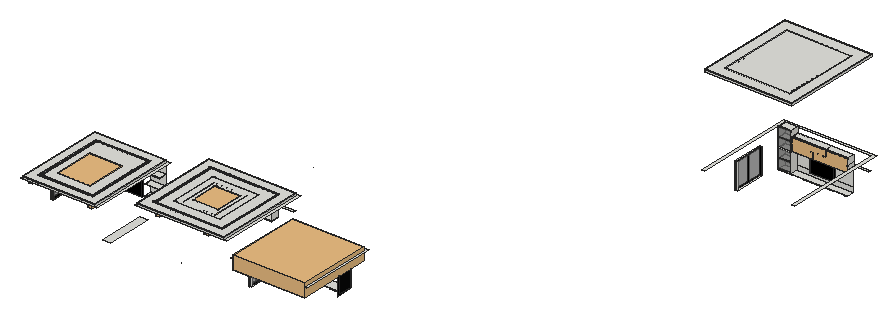
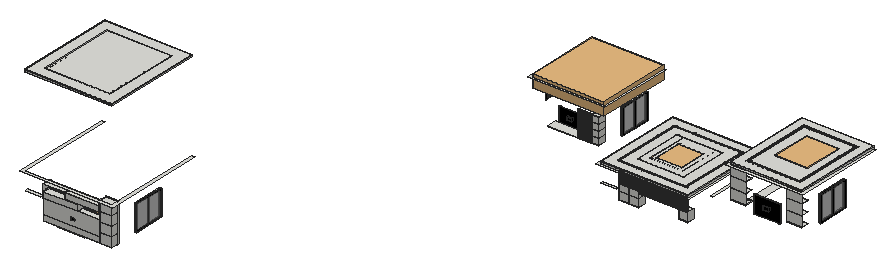
# SketchUp Ruby script. Lengths in inches.
U = 1.inch
M = Sketchup.active_model
def pt(a) = Geom::Point3d.new(a.map { |v| v * U })
def face(e, loops, mat)
  f = e.add_face(loops[0].map { |a| pt(a) })
  loops[1..].each { |l| e.add_face(l.map { |a| pt(a) }).erase! }
  f.material = f.back_material = mat if mat
  f
end
# faces: each face lists its corners as indices into pts; further lists are holes
def faces(e, pts, list, mat = nil) = list.each { |f| face(e, (f[0].is_a?(Array) ? f : [f]).map { |l| l.map { |i| pts[i] } }, mat) }
# xy, xz, yz: faces in a plane at the given z, y or x. An outline is a flat list of corners, or four numbers for a rectangle; further outlines are holes
def ring(l) = l.size == 4 ? [[l[0], l[1]], [l[2], l[1]], [l[2], l[3]], [l[0], l[3]]] : l.each_slice(2).to_a
def flat(e, list, mat, &to3) = list.each { |f| face(e, (f[0].is_a?(Array) ? f : [f]).map { |l| ring(l).map { |u, v| to3.(u, v) } }, mat) }
def xy(e, z, list, mat = nil) = flat(e, list, mat) { |x, y| [x, y, z] }
def xz(e, y, list, mat = nil) = flat(e, list, mat) { |x, z| [x, y, z] }
def yz(e, x, list, mat = nil) = flat(e, list, mat) { |y, z| [x, y, z] }
def lines(e, pts, list) = list.each { |a, b| e.add_line(pt(pts[a]), pt(pts[b])) }
# prism: a flat outline (further loops are holes) pulled along v
def prism(e, loops, v, mat = nil)
  f = face(e, loops, mat); d = Geom::Vector3d.new(v.map { |x| x * U })
  f.pushpull(f.normal.samedirection?(d) ? d.length : -d.length)
end
def box(e, o, s, mat = nil) = prism(e, [[o, [o[0] + s[0], o[1], o[2]], [o[0] + s[0], o[1] + s[1], o[2]], [o[0], o[1] + s[1], o[2]]]], [0, 0, s[2]], mat)
def at(x, y, z, deg = 0) = Geom::Transformation.translation(pt([x, y, z])) * Geom::Transformation.rotation(ORIGIN, Z_AXIS, deg.degrees)
def axes(o, x, y, z) = Geom::Transformation.new([*x, 0, *y, 0, *z, 0, *pt(o).to_a, 1])
def part(name) = M.definitions.add(name)
# library, detail: a bought-in or finely detailed component or shape, given as its bounding box
def library(name, o, s) = part(name).tap { |d| box(d.entities, o, s) }
def detail(e, o, s) = box(e.add_group.entities, o, s)
def put(e, d, t, mat = nil) = e.add_instance(d, t).tap { |i| i.material = mat if mat }
def group(e, t, mat = nil) = e.add_group.tap { |g| g.transformation = t; g.material = mat if mat }.entities
root = M.entities
M.materials.add("Chrome_Polished").color = [2, 2, 2]
M.materials.add("Plastic_Metalic_Black").color = [8, 8, 8]
M.materials.add("[0137_Black]").color = [0, 0, 0]
M.materials.add("[Color M00]1").color = [254, 254, 254]
M.materials.add("[Color_008]").color = [30, 30, 30]
M.materials.add("[Color_009]").color = [0, 0, 0]
M.materials.add("[Color_D14]").color = [173, 154, 131]
M.materials.add("[Translucent Glass Gray]1").color = [128, 128, 128]
M.materials["[Translucent Glass Gray]1"].alpha = 0.5
M.materials.add("[Translucent_Glass_Gray]").color = [128, 128, 128]
M.materials["[Translucent_Glass_Gray]"].alpha = 0.5
M.materials.add("blackened steel1").color = [30, 30, 30]
c1 = library("SKT_Nearly Natural 5' Kentia Palm Silk Tree",[-23.18,-17.61,0],[47.48,43.95,59.125])
c2 = part("Component\#22")
box(c2.entities,[0,-0.5,22.5],[28,0.5,21])
prism(c2.entities,[[[28,0,88],[28,0,77],[28,0,66.5],[0,0,66.5],[0,0,88]]],[0,-0.5,0])
prism(c2.entities,[[[0,0,44.5],[0,0,65.5],[28,0,65.5],[28,0,62],[28,0,47],[28,0,44.5]]],[0,-0.5,0])
box(c2.entities,[0,-0.5,0],[28,0.5,21.5])
c3 = part("Vertical wall batten \#3")
xy(c3.entities,0,[[0,-1,1,0]])
xy(c3.entities,60,[[0,-1,1,0]])
xz(c3.entities,-1,[[0,0,1,60]],"[Color_D14]")
xz(c3.entities,0,[[0,0,1,60]])
yz(c3.entities,0,[[-1,0,0,60]])
yz(c3.entities,1,[[-1,0,0,60]],"[Color_D14]")
c4 = part("Vertical wall batten \#1")
box(c4.entities,[0,-1,0],[1,1,30])
c5 = part("Photos Gallery Wall")
g1 = group(c5.entities,at(0,0,0))
xy(g1,23.66,[[13.71,0.34,13.7,1.03,31.9375,1.12,31.94,0.43]],"Plastic_Metalic_Black")
xy(g1,24.66,[[14.71,0.34,30.94,0.42,30.9375,1.02,14.7,0.94]],"Plastic_Metalic_Black")
xy(g1,48.82,[[14.71,0.34,14.7,0.94,30.9375,1.02,30.94,0.42]],"Plastic_Metalic_Black")
xy(g1,49.82,[[13.71,0.34,31.94,0.43,31.9375,1.12,13.7,1.03]],"Plastic_Metalic_Black")
p = [[13.7,1.03,49.82],[13.7,1.03,23.66],[13.71,0.34,23.66],[13.71,0.34,49.82],[31.94,0.43,23.66],[31.94,0.43,49.82],
  [30.94,0.42,24.66],[14.71,0.34,24.66],[14.71,0.34,48.82],[30.94,0.42,48.82],[31.9375,1.12,23.66],[31.9375,1.12,49.82],
  [14.7,1.04,24.66],[30.9375,1.11,24.66],[30.9375,1.11,48.82],[14.7,1.04,48.82],[14.7,0.94,48.82],[14.7,0.94,24.66],
  [30.9375,1.02,24.66],[30.9375,1.02,48.82],[29.9375,1.02,47.82],[29.9375,1.02,25.66],[15.7,0.95,25.66],[15.7,0.95,47.82]]
faces(g1,p,[[0,1,2,3],[[4,5,3,2],[6,7,8,9]],[10,11,5,4],[[11,10,1,0],[12,13,14,15]],[16,8,7,17],[18,6,9,19],[21,20,23,22]],"Plastic_Metalic_Black")
faces(g1,p,[[[17,18,19,16],[20,21,22,23]]],"[Color M00]1")
lines(g1,p,[[14,19],[15,16],[12,17],[13,18]])
c6 = part("Photo+Frames+03")
put(c6.entities,c5,axes([128.61,79.32,-32.19],[1.3608,0,0],[0,1.3608,0],[0,0,1.3608]))
c7 = part("Vertical wall batten \#2")
box(c7.entities,[0,-1,5],[1,1,25])
c8 = library("ceiling fan",[0,0,0],[76.25,93.13,30.02])
c9 = library("Group\#10",[-1.78,-1.38,0],[10.84,10.54,9.5])
c10 = part("Enscape.LinearLight")
xz(c10.entities,-59.06,[[0,-1,0,0,-0.38,-0.92],[0,-1,0.38,-0.92,0,0],[-0.38,-0.92,0,0,-0.71,-0.71],[0.38,-0.92,0.71,-0.71,0,0],[-0.71,-0.71,0,0,-0.92,-0.38],
  [0.71,-0.71,0.92,-0.38,0,0],[-0.92,-0.38,0,0,-1,0],[0.92,-0.38,1,0,0,0],[-1,0,0,0,-0.92,0.38],[0,0,-0.71,0.71,-0.92,0.38],
  [0,0,-0.38,0.92,-0.71,0.71],[0,0,0,1,-0.38,0.92],[0,0,0.38,0.92,0,1],[0,0,0.71,0.71,0.38,0.92],[0,0,0.92,0.38,0.71,0.71],
  [0,0,1,0,0.92,0.38]])
xz(c10.entities,59.06,[[0,-1,-0.38,-0.92,0,0],[0,-1,0,0,0.38,-0.92],[-0.38,-0.92,-0.71,-0.71,0,0],[0.38,-0.92,0,0,0.71,-0.71],[-0.71,-0.71,-0.92,-0.38,0,0],
  [0.71,-0.71,0,0,0.92,-0.38],[-0.92,-0.38,-1,0,0,0],[0.92,-0.38,0,0,1,0],[-1,0,-0.92,0.38,0,0],[0,0,-0.92,0.38,-0.71,0.71],
  [0,0,-0.71,0.71,-0.38,0.92],[0,0,-0.38,0.92,0,1],[0,0,0,1,0.38,0.92],[0,0,0.38,0.92,0.71,0.71],[0,0,0.71,0.71,0.92,0.38],
  [0,0,0.92,0.38,1,0]])
p = [[-0.38,-59.06,-0.92],[-0.38,59.06,-0.92],[0,59.06,-1],[0,-59.06,-1],[0.38,59.06,-0.92],[0.38,-59.06,-0.92],
  [-0.71,-59.06,-0.71],[-0.71,59.06,-0.71],[0.71,59.06,-0.71],[0.71,-59.06,-0.71],[-0.92,-59.06,-0.38],[-0.92,59.06,-0.38],
  [0.92,59.06,-0.38],[0.92,-59.06,-0.38],[-1,-59.06,0],[-1,59.06,0],[1,59.06,0],[1,-59.06,0],
  [-0.92,-59.06,0.38],[-0.92,59.06,0.38],[0.92,59.06,0.38],[0.92,-59.06,0.38],[-0.71,-59.06,0.71],[-0.71,59.06,0.71],
  [0.71,59.06,0.71],[0.71,-59.06,0.71],[-0.38,-59.06,0.92],[-0.38,59.06,0.92],[0.38,59.06,0.92],[0.38,-59.06,0.92],
  [0,-59.06,1],[0,59.06,1]]
faces(c10.entities,p,[[0,1,2],[0,2,3],[3,2,4],[3,4,5],[6,7,1],[6,1,0],[5,4,8],[5,8,9],
  [10,11,7],[10,7,6],[9,8,12],[9,12,13],[14,15,11],[14,11,10],[13,12,16],[13,16,17],
  [18,19,15],[18,15,14],[17,16,20],[17,20,21],[22,23,19],[22,19,18],[21,20,24],[21,24,25],
  [26,27,23],[26,23,22],[25,24,28],[25,28,29],[30,31,27],[30,27,26],[29,28,31],[29,31,30]])
c11 = part("Group\#11")
put(c11.entities,c10,at(1,59.06,1))
put(c11.entities,c10,at(1,102.94,1))
c12 = library("Group\#50",[0,0,0],[132,1,30])
c13 = library("Group\#24",[0,0,0],[168,174,30.02])
c14 = library("Group\#43",[-1.01,-0.93,0],[9.94,9.86,8.99])
c15 = part("Enscape.LinearLight\#2")
xz(c15.entities,-59.06,[[0,-1,0,0,-0.38,-0.92],[0,-1,0.38,-0.92,0,0],[-0.38,-0.92,0,0,-0.71,-0.71],[0.38,-0.92,0.71,-0.71,0,0],[-0.71,-0.71,0,0,-0.92,-0.38],
  [0.71,-0.71,0.92,-0.38,0,0],[-0.92,-0.38,0,0,-1,0],[0.92,-0.38,1,0,0,0],[-1,0,0,0,-0.92,0.38],[0,0,-0.71,0.71,-0.92,0.38],
  [0,0,-0.38,0.92,-0.71,0.71],[0,0,0,1,-0.38,0.92],[0,0,0.38,0.92,0,1],[0,0,0.71,0.71,0.38,0.92],[0,0,0.92,0.38,0.71,0.71],
  [0,0,1,0,0.92,0.38]])
xz(c15.entities,59.06,[[0,-1,-0.38,-0.92,0,0],[0,-1,0,0,0.38,-0.92],[-0.38,-0.92,-0.71,-0.71,0,0],[0.38,-0.92,0,0,0.71,-0.71],[-0.71,-0.71,-0.92,-0.38,0,0],
  [0.71,-0.71,0,0,0.92,-0.38],[-0.92,-0.38,-1,0,0,0],[0.92,-0.38,0,0,1,0],[-1,0,-0.92,0.38,0,0],[0,0,-0.92,0.38,-0.71,0.71],
  [0,0,-0.71,0.71,-0.38,0.92],[0,0,-0.38,0.92,0,1],[0,0,0,1,0.38,0.92],[0,0,0.38,0.92,0.71,0.71],[0,0,0.71,0.71,0.92,0.38],
  [0,0,0.92,0.38,1,0]])
p = [[-0.38,-59.06,-0.92],[-0.38,59.06,-0.92],[0,59.06,-1],[0,-59.06,-1],[0.38,59.06,-0.92],[0.38,-59.06,-0.92],
  [-0.71,-59.06,-0.71],[-0.71,59.06,-0.71],[0.71,59.06,-0.71],[0.71,-59.06,-0.71],[-0.92,-59.06,-0.38],[-0.92,59.06,-0.38],
  [0.92,59.06,-0.38],[0.92,-59.06,-0.38],[-1,-59.06,0],[-1,59.06,0],[1,59.06,0],[1,-59.06,0],
  [-0.92,-59.06,0.38],[-0.92,59.06,0.38],[0.92,59.06,0.38],[0.92,-59.06,0.38],[-0.71,-59.06,0.71],[-0.71,59.06,0.71],
  [0.71,59.06,0.71],[0.71,-59.06,0.71],[-0.38,-59.06,0.92],[-0.38,59.06,0.92],[0.38,59.06,0.92],[0.38,-59.06,0.92],
  [0,-59.06,1],[0,59.06,1]]
faces(c15.entities,p,[[0,1,2],[0,2,3],[3,2,4],[3,4,5],[6,7,1],[6,1,0],[5,4,8],[5,8,9],
  [10,11,7],[10,7,6],[9,8,12],[9,12,13],[14,15,11],[14,11,10],[13,12,16],[13,16,17],
  [18,19,15],[18,15,14],[17,16,20],[17,20,21],[22,23,19],[22,19,18],[21,20,24],[21,24,25],
  [26,27,23],[26,23,22],[25,24,28],[25,28,29],[30,31,27],[30,27,26],[29,28,31],[29,31,30]])
c16 = part("Group\#44")
put(c16.entities,c15,at(59.06,1,1,90))
put(c16.entities,c15,at(60.94,1,1,90))
c17 = part("Group\#45")
put(c17.entities,c16,at(2.29,42,0,90))
put(c17.entities,c16,at(2,0,0.0625,90))
xy(root,24,[[156.236,48,174.236,156]])
xy(root,25.053,[[309.446,291.299,331.946,309.299],[332.946,291.299,355.446,309.299]])
xy(root,26.053,[[309.446,291.299,331.946,309.299],[332.946,291.299,355.446,309.299]])
xy(root,28,[[1028.012,1017.859,1090.012,1033.859]])
xy(root,28.8,[[963.212,1017.859,994.812,1018.039],[995.212,1017.859,1026.812,1018.039],[1091.212,1017.859,1122.812,1018.039]])
xy(root,29,[[523.343,157.438,547.343,181.438],[548.343,157.438,598.343,181.438],[599.343,157.438,623.343,181.438],[963.012,1017.859,1027.012,1018.039],[1091.012,1017.859,1123.012,1018.039]])
xy(root,29.833,[[505.343,163.438,521.343,181.438]])
xy(root,30,[[522.343,157.438,624.343,181.438],[992.012,1017.859,1124.012,1033.859]])
xy(root,30.833,[[505.343,163.438,521.343,181.438]])
xy(root,31,[[963.012,1017.859,991.012,1035.859]])
xy(root,33.053,[[195.446,291.299,217.446,307.299]])
xy(root,34.053,[[195.446,291.299,217.446,307.299]])
xy(root,36,[[486.343,61.438,492.343,133.438],[0.236,90,6.236,162],[956.012,897.859,962.012,969.859]])
xy(root,43.053,[[309.446,291.299,331.946,309.299],[332.946,291.299,355.446,309.299]])
xy(root,44.053,[[309.446,291.299,331.946,309.299],[332.946,291.299,355.446,309.299]])
xy(root,44.5,[[505.343,163.438,521.343,181.438]])
xy(root,45.5,[[505.343,163.438,521.343,181.438]])
xy(root,46,[[6.236,192,42.236,210],[138.236,192,174.236,210]])
xy(root,47,[[6.236,192,42.236,210],[138.236,192,174.236,210]])
xy(root,49.553,[[356.446,309.299,392.446,315.299]])
xy(root,52.5,[[963.012,1017.859,991.012,1035.859]])
xy(root,53.5,[[963.012,1017.859,991.012,1035.859]])
xy(root,54.553,[[195.446,291.299,217.446,307.299]])
xy(root,55.553,[[194.446,291.299,218.446,309.299],[218.446,307.299,308.446,309.299]])
xy(root,59.167,[[505.343,163.438,521.343,181.438]])
xy(root,60.167,[[505.343,163.438,521.343,181.438]])
xy(root,60.553,[[309.446,291.299,331.946,309.299],[332.946,291.299,355.446,309.299]])
xy(root,61.553,[[188.446,147.299,194.446,243.299],[308.446,291.299,356.446,309.299]])
xy(root,70.5,[[6.236,192,42.236,210],[138.236,192,174.236,210]])
xy(root,71.5,[[6.236,192,42.236,210],[138.236,192,174.236,210]])
xy(root,73.833,[[505.343,163.438,521.343,181.438]])
xy(root,74.5,[[963.012,1017.859,991.012,1035.859]])
xy(root,74.833,[[505.343,163.438,521.343,181.438]])
xy(root,75.5,[[963.012,1017.859,991.012,1035.859]])
xy(root,78,[[1042.188,1018.859,1124.012,1033.859],[992.012,1019.039,1042.188,1033.859]])
xy(root,78.2,[[992.212,1018.859,1041.988,1019.039]])
xy(root,79,[[1043.188,1018.859,1123.012,1035.859]])
xy(root,84,[[1124.012,1035.859,1160.012,1041.859]])
xy(root,85.553,[[188.446,99.299,194.446,99.299,194.446,309.299,398.446,309.299,398.446,99.299,404.446,99.299,404.446,315.299,188.446,315.299]])
xy(root,89,[[505.343,163.438,521.343,181.438]])
xy(root,90,[[504.343,163.438,522.343,181.438]])
xy(root,92,[[1043.188,1018.859,1072.782,1035.859],[1072.782,1018.859,1123.012,1035.859]])
xy(root,92.8,[[992.212,1018.859,1041.988,1019.039]])
xy(root,93,[[992.012,1018.039,1042.188,1019.039],[1042.188,1018.039,1072.782,1018.859],[1072.782,1018.859,1124.012,1019.039]])
xy(root,93.2,[[1072.982,1018.859,1123.812,1019.039]])
xy(root,94,[[993.012,1018.039,1042.188,1035.859],[1042.188,1018.039,1071.782,1035.859]])
xy(root,95,[[6.236,192,42.236,210],[138.236,192,174.236,210]])
xy(root,96,[[486.343,61.438,492.343,133.438],[0.236,90,6.236,162],[6.236,192,42.236,210],[138.236,192,174.236,210],[956.012,897.859,962.012,969.859]])
xy(root,96.5,[[963.012,1017.859,991.012,1035.859]])
xy(root,97.5,[[963.012,1017.859,991.012,1035.859]])
xy(root,107,[[993.012,1018.039,1071.782,1035.859]])
xy(root,107.8,[[1072.982,1018.859,1123.812,1019.039]])
xy(root,108,[[992.012,1018.039,1072.782,1035.859],[1072.782,1019.039,1124.012,1035.859]])
xy(root,119,[[963.012,1017.859,991.012,1035.859]])
xy(root,120,[[0.236,0,6.236,0,6.236,210,174.236,210,174.236,0,180.236,0,180.236,216,0.236,216],[486.343,7.438,492.343,7.438,492.343,181.438,660.343,181.438,660.343,7.438,666.343,7.438,666.343,187.438,486.343,187.438],[956.012,801.859,962.012,801.859,962.012,1035.859,1166.012,1035.859,1166.012,801.859,1172.012,801.859,1172.012,1041.859,956.012,1041.859],[962.012,1017.859,992.012,1035.859]])
xz(root,61.438,[[486.343,36,492.343,96]])
xz(root,90,[[0.236,36,6.236,96]])
xz(root,133.438,[[486.343,36,492.343,96]])
xz(root,162,[[0.236,36,6.236,96]])
xz(root,181.438,[[505.343,30.833,521.343,44.5],[505.343,45.5,521.343,59.167],[505.343,60.167,521.343,73.833],[505.343,74.833,521.343,89]])
xz(root,192,[[6.236,46,42.236,47],[138.236,46,174.236,47],[6.236,70.5,42.236,71.5],[138.236,70.5,174.236,71.5],[6.236,95,42.236,96],
  [138.236,95,174.236,96]])
xz(root,210,[[6.236,47,42.236,70.5],[138.236,47,174.236,70.5],[6.236,71.5,42.236,95],[138.236,71.5,174.236,95],[6.236,96,42.236,120],
  [138.236,96,174.236,120]])
xz(root,307.299,[[195.446,34.053,217.446,54.553]])
xz(root,309.299,[[309.446,26.053,331.946,43.053],[332.946,26.053,355.446,43.053],[309.446,44.053,331.946,60.553],[332.946,44.053,355.446,60.553],[194.446,55.553,195.446,85.553]])
xz(root,897.859,[[956.012,36,962.012,96]])
xz(root,969.859,[[956.012,36,962.012,96]])
xz(root,1017.859,[[[962.012,30,992.012,120],[963.012,97.5,991.012,119],[963.012,31,991.012,52.5],[963.012,53.5,991.012,74.5],[963.012,75.5,991.012,96.5]]])
xz(root,1018.039,[[[992.012,93,1072.782,108],[993.012,94,1071.782,107]]],"blackened steel1")
xz(root,1018.859,[[992.212,78.2,1041.988,92.8],[1072.982,93.2,1123.812,107.8]])
xz(root,1018.859,[[[1042.188,78,1124.012,93],[1043.188,79,1123.012,92]]],"blackened steel1")
xz(root,1019.039,[[[992.012,78,1042.188,93],[992.212,78.2,1041.988,92.8]],[[1072.782,93,1124.012,108],[1072.982,93.2,1123.812,107.8]]],"blackened steel1")
xz(root,1033.859,[[992.012,30,1124.012,42],[992.012,42,1124.012,78]])
xz(root,1035.859,[[963.012,31,991.012,52.5],[963.012,53.5,991.012,74.5],[963.012,75.5,991.012,96.5],[1043.188,79,1123.012,92],[993.012,94,1071.782,107],
  [963.012,97.5,991.012,119]])
yz(root,42.236,[[192,46,210,47],[192,70.5,210,71.5],[192,95,210,96]])
yz(root,138.236,[[192,46,210,47],[192,70.5,210,71.5],[192,95,210,96]])
yz(root,195.446,[[291.299,34.053,307.299,54.553]])
yz(root,217.446,[[291.299,34.053,307.299,54.553]])
yz(root,309.446,[[291.299,26.053,309.299,43.053],[291.299,44.053,309.299,60.553]])
yz(root,331.946,[[291.299,26.053,309.299,43.053],[291.299,44.053,309.299,60.553]])
yz(root,332.946,[[291.299,26.053,309.299,43.053],[291.299,44.053,309.299,60.553]])
yz(root,355.446,[[291.299,26.053,309.299,43.053],[291.299,44.053,309.299,60.553]])
yz(root,505.343,[[163.438,30.833,181.438,44.5],[163.438,45.5,181.438,59.167],[163.438,60.167,181.438,73.833],[163.438,74.833,181.438,89]])
yz(root,521.343,[[163.438,30.833,181.438,44.5],[163.438,45.5,181.438,59.167],[163.438,60.167,181.438,73.833],[163.438,74.833,181.438,89]])
yz(root,522.343,[[163.438,30,181.438,90]])
yz(root,963.012,[[1017.859,31,1035.859,52.5],[1017.859,53.5,1035.859,74.5],[1017.859,75.5,1035.859,96.5],[1017.859,97.5,1035.859,119]])
yz(root,991.012,[[1017.859,31,1035.859,52.5],[1017.859,53.5,1035.859,74.5],[1017.859,75.5,1035.859,78],[1017.859,78,1035.859,93],[1017.859,93,1035.859,96.5],
  [1017.859,97.5,1035.859,108],[1017.859,108,1035.859,119]])
yz(root,992.012,[[1017.859,30,1033.859,78],[1017.859,78,1019.039,93],[1017.859,93,1018.039,108],[1017.859,108,1035.859,120]])
yz(root,992.212,[[1018.859,78.2,1019.039,92.8]])
yz(root,993.012,[[1018.039,94,1035.859,107]])
yz(root,1041.988,[[1018.859,78.2,1019.039,92.8]])
yz(root,1042.188,[[1018.859,78,1019.039,93]])
yz(root,1043.188,[[1018.859,79,1035.859,92]])
yz(root,1071.782,[[1018.039,94,1035.859,107]])
yz(root,1072.782,[[1018.039,93,1019.039,108]])
yz(root,1072.982,[[1018.859,93.2,1019.039,107.8]])
yz(root,1123.012,[[1018.859,79,1035.859,84],[1018.859,84,1035.859,92]])
yz(root,1123.812,[[1018.859,93.2,1019.039,107.8]])
yz(root,1124.012,[[1018.859,84,1035.859,93],[1019.039,93,1035.859,108]])
p = [[1256.272,-711.843,894.693],[1256.273,-711.843,894.693],[1256.273,-711.843,895.729],[1256.272,-711.843,895.729],[1114.607,-921.302,737.55],[1114.606,-921.302,737.55],
  [1114.606,-921.302,736.514],[1114.607,-921.302,736.514],[1041.611,-787.119,731.889],[1041.609,-787.118,731.889],[1041.609,-787.118,730.853],[1041.611,-787.119,730.853]]
lines(root,p,[[0,1],[2,3],[4,5],[6,7],[8,9],[10,11]])
put(root,c1,axes([531.29,163.12,29.99],[0.61,0,0],[0,0.61,0],[0,0,0.61]))
g2 = group(root,at(962.01,1016.86,30))
prism(g2,[[[30,1,0],[0,1,0],[0,1,90],[30,1,90],[30,1,78],[30,1,63],[30,1,48]],[[1,1,67.5],[29,1,67.5],[29,1,78],[29,1,89],[1,1,89]],[[1,1,22.5],[1,1,1],[29,1,1],[29,1,22.5]],[[1,1,23.5],[29,1,23.5],[29,1,44.5],[1,1,44.5]],[[29,1,45.5],[29,1,48],[29,1,63],[29,1,66.5],[1,1,66.5],[1,1,45.5]]],[0,-1,0])
put(g2,c2,at(1,1,1),"[Translucent Glass Gray]1")
put(root,c3,at(522.34,181.4375,30))
put(root,c3,at(523.54,181.4375,30))
put(root,c3,at(524.74,181.4375,30))
put(root,c3,at(525.94,181.4375,30))
put(root,c3,at(527.14,181.4375,30))
put(root,c3,at(528.34,181.4375,30))
put(root,c3,at(529.54,181.4375,30))
put(root,c3,at(530.74,181.4375,30))
put(root,c3,at(531.94,181.4375,30))
put(root,c3,at(533.14,181.4375,30))
put(root,c3,at(534.34,181.4375,30))
put(root,c3,at(535.54,181.4375,30))
put(root,c3,at(536.74,181.4375,30))
put(root,c3,at(537.94,181.4375,30))
put(root,c3,at(539.14,181.4375,30))
put(root,c3,at(540.34,181.4375,30))
put(root,c3,at(541.54,181.4375,30))
put(root,c3,at(542.74,181.4375,30))
put(root,c3,at(543.94,181.4375,30))
put(root,c3,at(545.14,181.4375,30))
put(root,c3,at(546.34,181.4375,30))
put(root,c3,at(547.54,181.4375,30))
put(root,c3,at(548.74,181.4375,30))
put(root,c3,at(549.94,181.4375,30))
put(root,c3,at(551.14,181.4375,30))
put(root,c3,at(552.34,181.4375,30))
g3 = group(root,at(122.4375,203.8125,32.2),"Chrome_Polished")
xy(g3,0,[[-62.2,0,0,2.1875]])
xy(g3,19.27,[[-37.69,2.1875,-24.125,5.1875]])
xy(g3,26.2,[[-37.69,2.1875,-24.125,5.1875]])
xy(g3,41.09,[[-62.2,0,0,2.1875]])
xz(g3,0,[[-62.2,0,0,41.09]])
xz(g3,2.1875,[[[-62.2,0,0,41.09],[-37.69,19.27,-24.125,26.2]]])
xz(g3,5.1875,[[-37.69,19.27,-24.125,26.2]])
yz(g3,-62.2,[[0,0,2.1875,41.09]])
yz(g3,-37.69,[[2.1875,19.27,5.1875,26.2]])
yz(g3,-24.125,[[2.1875,19.27,5.1875,26.2]])
yz(g3,0,[[0,0,2.1875,41.09]])
g4 = group(root,at(959.01,897.86,36))
xy(g4,0,[[-1.62,0,0,72]],"[Color_009]")
xy(g4,1.43,[[-1.62,1.71,-1.35,35.14],[-1.62,36.86,-1.35,70.29]])
xy(g4,1.43,[[-0.4,1.71,0,35.14],[-0.4,36.86,0,70.29]],"[Color_009]")
xy(g4,58.57,[[-1.62,1.71,-1.35,35.14],[-1.35,1.71,-0.4,35.14],[-0.4,1.71,0,35.14],[-1.62,36.86,-1.35,70.29],[-1.35,36.86,-0.4,70.29],
  [-0.4,36.86,0,70.29]])
xy(g4,60,[[-1.62,0,0,72]],"[Color_008]")
xz(g4,0,[[-1.62,0,0,60]],"[Color_009]")
xz(g4,1.71,[[-1.62,1.43,-1.35,58.57]])
xz(g4,1.71,[[-0.4,1.43,0,58.57]],"[Color_009]")
xz(g4,35.14,[[-1.62,1.43,-1.35,58.57],[-0.4,1.43,0,58.57]],"[Color_009]")
xz(g4,36.86,[[-1.62,1.43,-1.35,58.57],[-0.4,1.43,0,58.57]])
xz(g4,70.29,[[-1.62,1.43,-1.35,58.57],[-0.4,1.43,0,58.57]],"[Color_009]")
xz(g4,72,[[-1.62,0,0,60]],"[Color_009]")
yz(g4,-1.62,[[[0,0,72,60],[1.71,1.43,70.29,58.57]],[35.14,1.43,36.86,58.57]],"[Color_009]")
yz(g4,-1.35,[[1.71,1.43,35.14,58.57],[36.86,1.43,70.29,58.57]],"[Translucent_Glass_Gray]")
yz(g4,-0.4,[[1.71,1.43,35.14,58.57],[36.86,1.43,70.29,58.57]],"[Translucent_Glass_Gray]")
yz(g4,0,[[[0,0,72,60],[1.71,1.43,35.14,58.57],[36.86,1.43,70.29,58.57]]],"[Color_009]")
g5 = group(root,at(489.34,61.4375,36))
xy(g5,0,[[-2.74,0,0,72]],"[Color_009]")
xy(g5,1.43,[[-2.74,1.71,-2.28,35.14],[-2.74,36.86,-2.28,70.29]])
xy(g5,1.43,[[-0.69,1.71,0,35.14],[-0.69,36.86,0,70.29]],"[Color_009]")
xy(g5,58.57,[[-2.74,1.71,-2.28,35.14],[-2.28,1.71,-0.69,35.14],[-0.69,1.71,0,35.14],[-2.74,36.86,-2.28,70.29],[-2.28,36.86,-0.69,70.29],
  [-0.69,36.86,0,70.29]])
xy(g5,60,[[-2.74,0,0,72]],"[Color_008]")
xz(g5,0,[[-2.74,0,0,60]],"[Color_009]")
xz(g5,1.71,[[-2.74,1.43,-2.28,58.57]])
xz(g5,1.71,[[-0.69,1.43,0,58.57]],"[Color_009]")
xz(g5,35.14,[[-2.74,1.43,-2.28,58.57],[-0.69,1.43,0,58.57]],"[Color_009]")
xz(g5,36.86,[[-2.74,1.43,-2.28,58.57],[-0.69,1.43,0,58.57]])
xz(g5,70.29,[[-2.74,1.43,-2.28,58.57],[-0.69,1.43,0,58.57]],"[Color_009]")
xz(g5,72,[[-2.74,0,0,60]],"[Color_009]")
yz(g5,-2.74,[[[0,0,72,60],[1.71,1.43,70.29,58.57]],[35.14,1.43,36.86,58.57]],"[Color_009]")
yz(g5,-2.28,[[1.71,1.43,35.14,58.57],[36.86,1.43,70.29,58.57]],"[Translucent_Glass_Gray]")
yz(g5,-0.69,[[1.71,1.43,35.14,58.57],[36.86,1.43,70.29,58.57]],"[Translucent_Glass_Gray]")
yz(g5,0,[[[0,0,72,60],[1.71,1.43,35.14,58.57],[36.86,1.43,70.29,58.57]]],"[Color_009]")
g6 = group(root,at(3.24,90,36))
xy(g6,0,[[-3.24,0,0,72]],"[Color_009]")
xy(g6,1.43,[[-3.24,1.71,-2.7,35.14],[-3.24,36.86,-2.7,70.29]])
xy(g6,1.43,[[-0.81,1.71,0,35.14],[-0.81,36.86,0,70.29]],"[Color_009]")
xy(g6,58.57,[[-3.24,1.71,-2.7,35.14],[-2.7,1.71,-0.81,35.14],[-0.81,1.71,0,35.14],[-3.24,36.86,-2.7,70.29],[-2.7,36.86,-0.81,70.29],
  [-0.81,36.86,0,70.29]])
xy(g6,60,[[-3.24,0,0,72]],"[Color_008]")
xz(g6,0,[[-3.24,0,0,60]],"[Color_009]")
xz(g6,1.71,[[-3.24,1.43,-2.7,58.57]])
xz(g6,1.71,[[-0.81,1.43,0,58.57]],"[Color_009]")
xz(g6,35.14,[[-3.24,1.43,-2.7,58.57],[-0.81,1.43,0,58.57]],"[Color_009]")
xz(g6,36.86,[[-3.24,1.43,-2.7,58.57],[-0.81,1.43,0,58.57]])
xz(g6,70.29,[[-3.24,1.43,-2.7,58.57],[-0.81,1.43,0,58.57]],"[Color_009]")
xz(g6,72,[[-3.24,0,0,60]],"[Color_009]")
yz(g6,-3.24,[[[0,0,72,60],[1.71,1.43,70.29,58.57]],[35.14,1.43,36.86,58.57]],"[Color_009]")
yz(g6,-2.7,[[1.71,1.43,35.14,58.57],[36.86,1.43,70.29,58.57]],"[Translucent_Glass_Gray]")
yz(g6,-0.81,[[1.71,1.43,35.14,58.57],[36.86,1.43,70.29,58.57]],"[Translucent_Glass_Gray]")
yz(g6,0,[[[0,0,72,60],[1.71,1.43,35.14,58.57],[36.86,1.43,70.29,58.57]]],"[Color_009]")
g7 = group(root,at(1083.3,1028.86,38.98),"[0137_Black]")
xy(g7,0,[[-55.82,0,0,2]])
xy(g7,15.29,[[-31.67,2,-23.58,5]])
xy(g7,20.29,[[-31.67,2,-23.58,5]])
xy(g7,34.5,[[-55.82,0,0,2]])
xz(g7,0,[[-55.82,0,0,34.5]])
xz(g7,2,[[[-55.82,0,0,34.5],[-31.67,15.29,-23.58,20.29]]])
xz(g7,5,[[-31.67,15.29,-23.58,20.29]])
yz(g7,-55.82,[[0,0,2,34.5]])
yz(g7,-31.67,[[2,15.29,5,20.29]])
yz(g7,-23.58,[[2,15.29,5,20.29]])
yz(g7,0,[[0,0,2,34.5]])
g8 = group(root,at(602.65,175.4375,43.4375),"[0137_Black]")
xy(g8,0,[[-54.1,0,0,2]])
xy(g8,13.83,[[-34.28,2,-21.78,5]])
xy(g8,20.58,[[-34.28,2,-21.78,5]])
xy(g8,33.4375,[[-54.1,0,0,2]])
xz(g8,0,[[-54.1,0,0,33.4375]])
xz(g8,2,[[[-54.1,0,0,33.4375],[-34.28,13.83,-21.78,20.58]]])
xz(g8,5,[[-34.28,13.83,-21.78,20.58]])
yz(g8,-54.1,[[0,0,2,33.4375]])
yz(g8,-34.28,[[2,13.83,5,20.58]])
yz(g8,-21.78,[[2,13.83,5,20.58]])
yz(g8,0,[[0,0,2,33.4375]])
put(root,c4,at(194.45,309.3,55.55))
put(root,c4,at(195.65,309.3,55.55))
put(root,c4,at(196.85,309.3,55.55))
put(root,c4,at(198.05,309.3,55.55))
put(root,c4,at(199.25,309.3,55.55))
put(root,c4,at(200.45,309.3,55.55))
put(root,c4,at(201.65,309.3,55.55))
put(root,c4,at(202.85,309.3,55.55))
put(root,c4,at(204.05,309.3,55.55))
put(root,c4,at(205.25,309.3,55.55))
put(root,c4,at(206.45,309.3,55.55))
put(root,c4,at(207.65,309.3,55.55))
put(root,c4,at(208.85,309.3,55.55))
put(root,c4,at(210.05,309.3,55.55))
put(root,c4,at(211.25,309.3,55.55))
put(root,c4,at(212.45,309.3,55.55))
put(root,c4,at(213.65,309.3,55.55))
put(root,c4,at(214.85,309.3,55.55))
put(root,c4,at(216.05,309.3,55.55))
put(root,c4,at(217.25,309.3,55.55))
put(root,c4,at(218.45,309.3,55.55))
put(root,c4,at(219.65,309.3,55.55))
put(root,c4,at(220.85,309.3,55.55))
put(root,c4,at(222.05,309.3,55.55))
put(root,c4,at(223.25,309.3,55.55))
put(root,c4,at(224.45,309.3,55.55))
put(root,c4,at(225.65,309.3,55.55))
put(root,c4,at(226.85,309.3,55.55))
put(root,c4,at(228.05,309.3,55.55))
put(root,c4,at(229.25,309.3,55.55))
put(root,c4,at(230.45,309.3,55.55))
put(root,c4,at(231.65,309.3,55.55))
put(root,c4,at(232.85,309.3,55.55))
put(root,c4,at(234.05,309.3,55.55))
put(root,c4,at(235.25,309.3,55.55))
put(root,c4,at(236.45,309.3,55.55))
put(root,c4,at(237.65,309.3,55.55))
put(root,c4,at(238.85,309.3,55.55))
put(root,c4,at(240.05,309.3,55.55))
put(root,c4,at(241.25,309.3,55.55))
put(root,c4,at(242.45,309.3,55.55))
put(root,c4,at(243.65,309.3,55.55))
put(root,c4,at(244.85,309.3,55.55))
put(root,c4,at(246.05,309.3,55.55))
put(root,c4,at(247.25,309.3,55.55))
put(root,c4,at(248.45,309.3,55.55))
put(root,c4,at(249.65,309.3,55.55))
put(root,c4,at(250.85,309.3,55.55))
put(root,c4,at(252.05,309.3,55.55))
put(root,c4,at(253.25,309.3,55.55))
put(root,c4,at(254.45,309.3,55.55))
put(root,c4,at(255.65,309.3,55.55))
put(root,c4,at(256.85,309.3,55.55))
put(root,c4,at(258.05,309.3,55.55))
put(root,c4,at(259.25,309.3,55.55))
put(root,c4,at(260.45,309.3,55.55))
put(root,c4,at(261.65,309.3,55.55))
put(root,c4,at(262.85,309.3,55.55))
put(root,c4,at(264.05,309.3,55.55))
put(root,c4,at(265.25,309.3,55.55))
put(root,c4,at(266.45,309.3,55.55))
put(root,c4,at(267.65,309.3,55.55))
put(root,c4,at(268.85,309.3,55.55))
put(root,c4,at(270.05,309.3,55.55))
put(root,c4,at(271.25,309.3,55.55))
put(root,c4,at(272.45,309.3,55.55))
put(root,c4,at(273.65,309.3,55.55))
put(root,c4,at(274.85,309.3,55.55))
put(root,c4,at(276.05,309.3,55.55))
put(root,c4,at(277.25,309.3,55.55))
put(root,c4,at(278.45,309.3,55.55))
put(root,c4,at(279.65,309.3,55.55))
put(root,c4,at(280.85,309.3,55.55))
put(root,c4,at(282.05,309.3,55.55))
put(root,c4,at(283.25,309.3,55.55))
put(root,c4,at(284.45,309.3,55.55))
put(root,c4,at(285.65,309.3,55.55))
put(root,c4,at(286.85,309.3,55.55))
put(root,c4,at(288.05,309.3,55.55))
put(root,c4,at(289.25,309.3,55.55))
put(root,c4,at(290.45,309.3,55.55))
put(root,c4,at(291.65,309.3,55.55))
put(root,c4,at(292.85,309.3,55.55))
put(root,c4,at(294.05,309.3,55.55))
put(root,c4,at(295.25,309.3,55.55))
put(root,c4,at(296.45,309.3,55.55))
put(root,c4,at(297.65,309.3,55.55))
put(root,c4,at(298.85,309.3,55.55))
put(root,c4,at(300.05,309.3,55.55))
put(root,c4,at(301.25,309.3,55.55))
put(root,c4,at(302.45,309.3,55.55))
put(root,c4,at(303.65,309.3,55.55))
put(root,c4,at(304.85,309.3,55.55))
put(root,c4,at(306.05,309.3,55.55))
put(root,c4,at(307.25,309.3,55.55))
put(root,c4,at(308.45,309.3,55.55))
put(root,c6,axes([579.5,373.86,56.25],[0,-1.56,0],[1,0,0],[0,0,1.26]))
put(root,c7,at(309.65,309.3,55.55))
put(root,c7,at(310.85,309.3,55.55))
put(root,c7,at(312.05,309.3,55.55))
put(root,c7,at(313.25,309.3,55.55))
put(root,c7,at(314.45,309.3,55.55))
put(root,c7,at(315.65,309.3,55.55))
put(root,c7,at(316.85,309.3,55.55))
put(root,c7,at(318.05,309.3,55.55))
put(root,c7,at(319.25,309.3,55.55))
put(root,c7,at(320.45,309.3,55.55))
put(root,c7,at(321.65,309.3,55.55))
put(root,c7,at(322.85,309.3,55.55))
put(root,c7,at(324.05,309.3,55.55))
put(root,c7,at(325.25,309.3,55.55))
put(root,c7,at(326.45,309.3,55.55))
put(root,c7,at(327.65,309.3,55.55))
put(root,c7,at(328.85,309.3,55.55))
put(root,c7,at(330.05,309.3,55.55))
put(root,c7,at(331.25,309.3,55.55))
put(root,c7,at(332.45,309.3,55.55))
put(root,c7,at(333.65,309.3,55.55))
put(root,c7,at(334.85,309.3,55.55))
put(root,c7,at(336.05,309.3,55.55))
put(root,c7,at(337.25,309.3,55.55))
put(root,c7,at(338.45,309.3,55.55))
put(root,c7,at(339.65,309.3,55.55))
put(root,c7,at(340.85,309.3,55.55))
put(root,c7,at(342.05,309.3,55.55))
put(root,c7,at(343.25,309.3,55.55))
put(root,c7,at(344.45,309.3,55.55))
put(root,c7,at(345.65,309.3,55.55))
put(root,c7,at(346.85,309.3,55.55))
put(root,c7,at(348.05,309.3,55.55))
put(root,c7,at(349.25,309.3,55.55))
put(root,c7,at(350.45,309.3,55.55))
put(root,c7,at(351.65,309.3,55.55))
put(root,c7,at(352.85,309.3,55.55))
put(root,c7,at(354.05,309.3,55.55))
put(root,c7,at(355.25,309.3,55.55))
g9 = group(root,at(194.45,99.3,64.32))
xy(g9,21.24,[[[0,0,204,210],[24,24,180,186]]])
xy(g9,25.24,[[[0,0,204,210],[22,22,182,188]],[22,22,180,24],[180,22,182,188],[22,24,24,186],[22,186,180,188]])
xy(g9,27.24,[[[0,0,204,210],[22,22,182,188]],[[22,22,182,188],[48,48,156,162]],[72,72,132,138]])
xy(g9,28.24,[[[48,48,156,162],[72,72,132,138]]])
xz(g9,0,[[0,21.24,204,25.24],[0,25.24,204,27.24]])
xz(g9,22,[[22,25.24,182,27.24]])
xz(g9,24,[[24,21.24,180,25.24]])
xz(g9,48,[[48,27.24,156,28.24]])
xz(g9,72,[[72,27.24,132,28.24]])
xz(g9,138,[[72,27.24,132,28.24]])
xz(g9,162,[[48,27.24,156,28.24]])
xz(g9,186,[[24,21.24,180,25.24]])
xz(g9,188,[[22,25.24,182,27.24]])
xz(g9,210,[[0,21.24,1,25.24],[1,21.24,204,25.24],[0,25.24,1,27.24],[1,25.24,204,27.24]])
yz(g9,0,[[0,21.24,210,25.24],[0,25.24,210,27.24]])
yz(g9,22,[[22,25.24,188,27.24]])
yz(g9,24,[[24,21.24,186,25.24]])
yz(g9,48,[[48,27.24,162,28.24]])
yz(g9,72,[[72,27.24,138,28.24]])
yz(g9,132,[[72,27.24,138,28.24]])
yz(g9,156,[[48,27.24,162,28.24]])
yz(g9,180,[[24,21.24,186,25.24]])
yz(g9,182,[[22,25.24,188,27.24]])
yz(g9,204,[[0,21.24,210,25.24],[0,25.24,210,27.24]])
put(g9,c8,axes([63.66,52.66,0],[1,0,0],[0,1,0],[0,0,0.92]))
put(g9,c9,axes([18.1,44.22,21.24],[-1,0,0],[0,1,0],[0,0,-1]))
put(g9,c9,axes([159.9375,7.73,21.24],[-1,0,0],[0,1,0],[0,0,-1]))
put(g9,c9,axes([159.9375,193.1,21.24],[-1,0,0],[0,1,0],[0,0,-1]))
put(g9,c9,axes([194.85,44.22,21.24],[-1,0,0],[0,1,0],[0,0,-1]))
put(g9,c9,axes([47.125,7.73,21.24],[-1,0,0],[0,1,0],[0,0,-1]))
put(g9,c9,axes([47.125,193.1,21.24],[-1,0,0],[0,1,0],[0,0,-1]))
put(g9,c9,axes([18.1,156.34,21.24],[-1,0,0],[0,1,0],[0,0,-1]))
put(g9,c9,axes([194.85,156.34,21.24],[-1,0,0],[0,1,0],[0,0,-1]))
put(g9,c11,at(18,24,25.24,-90))
put(g9,c11,at(180,24,25.24))
put(g9,c11,at(18,188,25.24,-90))
put(g9,c11,at(22,24,25.24))
put(root,c12,at(992.01,1017.86,78))
put(root,c13,at(492.34,7.4375,97.1))
g10 = group(root,at(6.24,0,98.69))
put(g10,c8,axes([42.52,48.67,0],[1,0,0],[0,1,0],[0,0,0.91]))
g11 = group(g10,at(0,0,27.31))
xy(g11,-6,[[[0,0,168,210],[24,24,144,186]]])
xy(g11,-2,[[[0,0,168,210],[20,20,148,190]],[20,20,24,190],[24,20,144,24],[144,20,148,190],[24,186,144,190]])
xy(g11,0,[[[0,0,168,210],[20,20,148,190]],[20,20,148,190]])
xz(g11,0,[[0,-6,168,-2],[0,-2,168,0]])
xz(g11,20,[[20,-2,148,0]])
xz(g11,24,[[24,-6,144,-2]])
xz(g11,186,[[24,-6,144,-2]])
xz(g11,190,[[20,-2,148,0]])
xz(g11,210,[[0,-6,168,-2],[0,-2,168,0]])
yz(g11,0,[[0,-6,210,-2],[0,-2,210,0]])
yz(g11,20,[[20,-2,190,0]])
yz(g11,24,[[24,-6,186,-2]])
yz(g11,144,[[24,-6,186,-2]])
yz(g11,148,[[20,-2,190,0]])
yz(g11,168,[[0,-6,210,-2],[0,-2,210,0]])
put(g11,c14,axes([16.75,9.01,-6],[-1,0,0],[0,1,0],[0,0,-1]))
put(g11,c14,axes([157.89,5.59,-6],[-1,0,0],[0,1,0],[0,0,-1]))
put(g11,c14,axes([16.75,196.26,-6],[-1,0,0],[0,1,0],[0,0,-1]))
put(g11,c14,axes([157.89,192.84,-6],[-1,0,0],[0,1,0],[0,0,-1]))
put(g11,c14,axes([16.75,68.44,-6],[-1,0,0],[0,1,0],[0,0,-1]))
put(g11,c14,axes([157.89,65.03,-6],[-1,0,0],[0,1,0],[0,0,-1]))
put(g11,c14,axes([16.75,130.19,-6],[-1,0,0],[0,1,0],[0,0,-1]))
put(g11,c14,axes([157.89,126.78,-6],[-1,0,0],[0,1,0],[0,0,-1]))
put(g10,c16,at(24,185.71,25.02))
put(g10,c17,at(144,24,25.31))
put(g10,c17,at(22,24,25.25))
put(g10,c16,at(24,22,25.31))
g12 = group(root,at(962.01,801.86,333.5))
xy(g12,-6,[[[0,0,204,234],[30,30,174,204]]])
xy(g12,-2,[[[0,0,204,234],[26,26,178,208]],[26,26,178,30],[26,30,30,204],[174,30,178,204],[26,204,178,208]])
xy(g12,0,[[[0,0,204,234],[26,26,178,208]],[26,26,178,208]])
xz(g12,0,[[0,-6,204,-2],[0,-2,204,0]])
xz(g12,26,[[26,-2,178,0]])
xz(g12,30,[[30,-6,174,-2]])
xz(g12,204,[[30,-6,174,-2]])
xz(g12,208,[[26,-2,178,0]])
xz(g12,234,[[0,-6,204,-2],[0,-2,204,0]])
yz(g12,0,[[0,-6,234,-2],[0,-2,234,0]])
yz(g12,26,[[26,-2,208,0]])
yz(g12,30,[[30,-6,204,-2]])
yz(g12,174,[[30,-6,204,-2]])
yz(g12,178,[[26,-2,208,0]])
yz(g12,204,[[0,-6,234,-2],[0,-2,234,0]])
